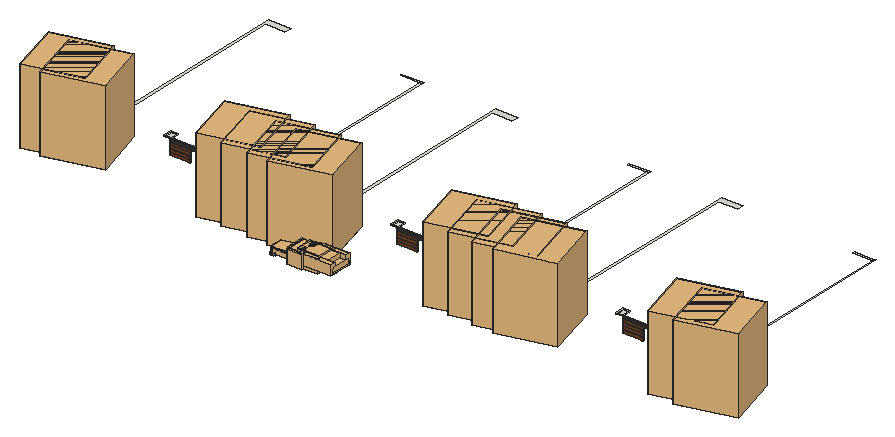
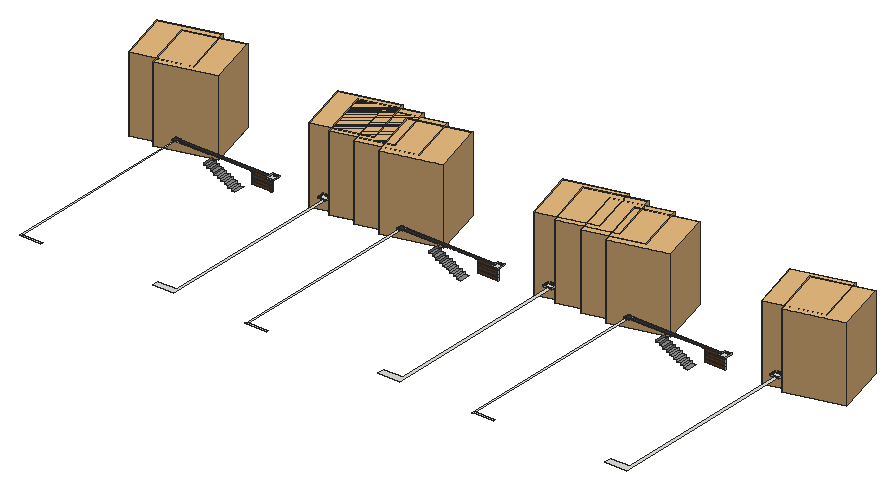
# SketchUp Ruby script. Lengths in inches.
U = 1.inch
M = Sketchup.active_model
def pt(a) = Geom::Point3d.new(a.map { |v| v * U })
def face(e, loops, mat)
  f = e.add_face(loops[0].map { |a| pt(a) })
  loops[1..].each { |l| e.add_face(l.map { |a| pt(a) }).erase! }
  f.material = f.back_material = mat if mat
  f
end
# faces: each face lists its corners as indices into pts; further lists are holes
def faces(e, pts, list, mat = nil) = list.each { |f| face(e, (f[0].is_a?(Array) ? f : [f]).map { |l| l.map { |i| pts[i] } }, mat) }
# xy, xz, yz: faces in a plane at the given z, y or x. An outline is a flat list of corners, or four numbers for a rectangle; further outlines are holes
def ring(l) = l.size == 4 ? [[l[0], l[1]], [l[2], l[1]], [l[2], l[3]], [l[0], l[3]]] : l.each_slice(2).to_a
def flat(e, list, mat, &to3) = list.each { |f| face(e, (f[0].is_a?(Array) ? f : [f]).map { |l| ring(l).map { |u, v| to3.(u, v) } }, mat) }
def xy(e, z, list, mat = nil) = flat(e, list, mat) { |x, y| [x, y, z] }
def xz(e, y, list, mat = nil) = flat(e, list, mat) { |x, z| [x, y, z] }
def yz(e, x, list, mat = nil) = flat(e, list, mat) { |y, z| [x, y, z] }
def lines(e, pts, list) = list.each { |a, b| e.add_line(pt(pts[a]), pt(pts[b])) }
# prism: a flat outline (further loops are holes) pulled along v
def prism(e, loops, v, mat = nil)
  f = face(e, loops, mat); d = Geom::Vector3d.new(v.map { |x| x * U })
  f.pushpull(f.normal.samedirection?(d) ? d.length : -d.length)
end
def box(e, o, s, mat = nil) = prism(e, [[o, [o[0] + s[0], o[1], o[2]], [o[0] + s[0], o[1] + s[1], o[2]], [o[0], o[1] + s[1], o[2]]]], [0, 0, s[2]], mat)
def at(x, y, z, deg = 0) = Geom::Transformation.translation(pt([x, y, z])) * Geom::Transformation.rotation(ORIGIN, Z_AXIS, deg.degrees)
def axes(o, x, y, z) = Geom::Transformation.new([*x, 0, *y, 0, *z, 0, *pt(o).to_a, 1])
def part(name) = M.definitions.add(name)
# library, detail: a bought-in or finely detailed component or shape, given as its bounding box
def library(name, o, s) = part(name).tap { |d| box(d.entities, o, s) }
def detail(e, o, s) = box(e.add_group.entities, o, s)
def put(e, d, t, mat = nil) = e.add_instance(d, t).tap { |i| i.material = mat if mat }
def group(e, t, mat = nil) = e.add_group.tap { |g| g.transformation = t; g.material = mat if mat }.entities
root = M.entities
M.materials.add("[0132_LightGray]").color = [169, 169, 169]
M.materials.add("[0136_Charcoal]").color = [17, 17, 17]
M.materials.add("[Blacktop Old 02]").color = [143, 145, 145]
M.materials.add("[Color M07]").color = [58, 58, 58]
M.materials.add("[Wood Veneer 01]").color = [120, 70, 37]
M.materials.add("s500 white").color = [237, 237, 230]
M.materials.add("s600").color = [22, 22, 22]
c1 = library("Group\#538",[0,0,0],[7.9,66.99,3.86])
c2 = library("Front car door",[0,0,0],[50.01,18.32,46.37])
c3 = library("Rear car door",[0,0,0],[51.74,11.92,46.37])
c4 = library("Palm tree \#1",[-4.09,-4.52,0],[193.52,193.51,258.93])
c5 = part("Palm+Tree")
put(c5.entities,c4,at(25.51,-21.81,0,15))
c6 = library("Group\#523",[0,0,0],[21.93,78.33,4.58])
c7 = library("Group\#520",[0,0,0],[63.89,71.13,20.26])
c8 = part("Group\#531")
p = [[17.05,0,0.12],[10.76,0.83,0.14],[10.77,0.78,0],[8.125,1.26,0.14],[7.82,1.25,0],[5.66,2.14,0],
  [5.93,2.16,0.13],[4.78,3.14,0.17],[4.32,3.23,0],[3.41,4.89,0],[3.73,4.98,0.17],[1.67,12.39,0],
  [2,12.39,0.17],[0,22.05,0],[0.34,21.8125,0.17],[1.49,22.05,0.22],[16.1,0.375,0.31],[17.15,0.01,0.31],
  [14.125,0.92,0.31],[11.23,1.28,0.31],[8.51,1.62,0.31],[5.54,2.89,0.31],[5.22,3.53,0.31],[4.82,5.07,0.31],
  [3.125,12.39,0.31],[1.65,21.85,0.31]]
faces(c8.entities,p,[[0,1,2],[2,3,4],[3,2,1],[5,4,6],[6,4,3],[7,8,5],[7,5,6],[9,7,10],
  [7,9,8],[11,9,12],[12,9,10],[13,11,14],[14,11,12],[14,15,13],[16,1,17],[1,0,17],
  [1,16,18],[19,3,1],[19,1,18],[3,20,6],[3,19,20],[6,20,21],[21,7,6],[22,7,21],
  [10,7,23],[22,23,7],[24,12,10],[23,24,10],[14,12,25],[24,25,12],[14,25,15]],"[0132_LightGray]")
c9 = library("Group\#541",[0,74.4,0],[63.33,6.34,17.85])
c10 = library("Component\#24",[0,0,0],[112.42,14.7,36.85])
c11 = library("Car headlight",[-0.14,0,-0.04],[12.61,20.03,8.76])
c12 = library("Group\#517",[0,0,0],[9.48,71.95,2.68])
c13 = library("Group\#529",[0,0,0],[27.27,66.27,16.46])
c14 = library("Group\#527",[0,0,0],[8.93,15.28,7.15])
c15 = library("Group\#519",[0,0,0],[35.29,74.27,19.26])
c16 = library("Group\#535",[-5.26,0,0],[129.69,69.79,18.37])
c17 = part("3D_Object__24")
g1 = group(c17.entities,at(-0.5,-39.39,30.52))
p = [[0.5,0,0],[0.5,0.09,0.49],[0.27,0.1875,0.49],[0.15,0.15,0.01],[0.85,0.15,0.01],[0.73,0.1875,0.49],
  [0.18,0.41,0.5],[0,0.5,0.02],[1,0.5,0.02],[0.82,0.41,0.5],[0.27,0.64,0.51],[0.15,0.85,0.04],
  [0.85,0.85,0.04],[0.73,0.64,0.51],[0.5,0.73,0.52],[0.5,1,0.04],[0.5,0.1,0.9],[0.33,0.17,0.9],
  [0.67,0.17,0.9],[0.26,0.34,0.91],[0.74,0.34,0.91],[0.33,0.5,0.91],[0.67,0.5,0.91],[0.5,0.57,0.91],
  [0.34,0.09,1.16],[0.5,0.03,1.16],[0.5,0.24,1.22],[0.66,0.09,1.16],[0.27,0.26,1.17],[0.73,0.26,1.17],
  [0.34,0.42,1.17],[0.5,0.48,1.17],[0.66,0.42,1.17]]
faces(g1,p,[[0,1,2,3],[4,5,1,0],[3,2,6,7],[8,9,5,4],[7,6,10,11],[12,13,9,8],[11,10,14,15],[15,14,13,12],
  [1,16,17,2],[1,5,18,16],[6,2,19],[17,19,2],[9,20,5],[18,5,20],[19,21,6],[20,9,22],
  [10,6,21],[13,22,9],[10,21,14],[23,14,21],[13,14,22],[23,22,14],[24,25,26],[25,27,26],
  [28,24,26],[27,29,26],[30,28,26],[31,30,26],[32,31,26],[29,32,26]])
g2 = group(c17.entities,at(-0.24,-39.37,31.42))
p = [[0.24,0.08,0],[0.24,0,0.26],[0.07,0.07,0.26],[0.07,0.14,0],[0.4,0.14,0],[0.4,0.07,0.26],
  [0.01,0.23,0.27],[0,0.31,0.01],[0.47,0.31,0.01],[0.46,0.23,0.27],[0.07,0.39,0.27],[0.07,0.48,0.01],
  [0.4,0.48,0.01],[0.4,0.39,0.27],[0.24,0.46,0.27],[0.24,0.54,0.01]]
faces(g2,p,[[0,1,2,3],[4,5,1,0],[3,2,6,7],[8,9,5,4],[7,6,10,11],[12,13,9,8],[11,10,14,15],[15,14,13,12]],"[0132_LightGray]")
c18 = library("Group\#540",[0,0,0],[73.87,53.92,3.7])
xy(root,13.04,[[998.26,300.25,1070.49,301],[1784.63,300.25,1856.87,301],[2565.01,300.25,2637.24,301]])
xy(root,17.875,[[1073.03,335.33,1085.03,371.33],[1859.4,335.33,1871.4,371.33],[2639.78,335.33,2651.78,371.33]],"[Blacktop Old 02]")
xy(root,22.41,[[998.26,300.25,1070.49,301],[1784.63,300.25,1856.87,301],[2565.01,300.25,2637.24,301]])
xy(root,23.79,[[998.26,300.25,1070.49,301],[1784.63,300.25,1856.87,301],[2565.01,300.25,2637.24,301]])
xy(root,23.875,[[1085.03,335.33,1097.03,371.33],[1871.4,335.33,1883.4,371.33],[2651.78,335.33,2663.78,371.33]],"[Blacktop Old 02]")
xy(root,29.875,[[1097.03,335.33,1109.03,371.33],[1883.4,335.33,1895.4,371.33],[2663.78,335.33,2675.78,371.33]],"[Blacktop Old 02]")
xy(root,33.16,[[998.26,300.25,1070.49,301],[1784.63,300.25,1856.87,301],[2565.01,300.25,2637.24,301]])
xy(root,34.54,[[998.26,300.25,1070.49,301],[1784.63,300.25,1856.87,301],[2565.01,300.25,2637.24,301]])
xy(root,35.875,[[1109.03,335.33,1121.03,371.33],[1895.4,335.33,1907.4,371.33],[2675.78,335.33,2687.78,371.33]],"[Blacktop Old 02]")
xy(root,41.875,[[1121.03,335.33,1133.03,371.33],[1907.4,335.33,1919.4,371.33],[2687.78,335.33,2699.78,371.33]],"[Blacktop Old 02]")
xy(root,43.91,[[998.26,300.25,1070.49,301],[1784.63,300.25,1856.87,301],[2565.01,300.25,2637.24,301]])
xy(root,45.29,[[998.26,300.25,1070.49,301],[1784.63,300.25,1856.87,301],[2565.01,300.25,2637.24,301]])
xy(root,47.875,[[1133.03,335.33,1145.03,371.33],[1919.4,335.33,1931.4,371.33],[2699.78,335.33,2711.78,371.33]],"[Blacktop Old 02]")
xy(root,53.875,[[1145.03,335.33,1157.03,371.33],[1931.4,335.33,1943.4,371.33],[2711.78,335.33,2723.78,371.33]],"[Blacktop Old 02]")
xy(root,54.66,[[1070.49,300.25,1216.78,301],[1219.26,300.25,1219.97,301],[1222.44,300.25,1223.16,301],[1225.63,300.25,1226.35,301],[1228.82,300.25,1229.53,301],
  [1232.01,300.25,1232.72,301],[1235.19,300.25,1235.91,301],[1238.38,300.25,1239.1,301],[1241.57,300.25,1242.28,301],[1244.76,300.25,1245.47,301],
  [1247.94,300.25,1248.66,301],[1251.13,300.25,1251.85,301],[1254.32,300.25,1255.03,301],[1257.51,300.25,1258.22,301],[1260.69,300.25,1261.41,301],
  [1263.88,300.25,1264.6,301],[1267.07,300.25,1267.78,301],[1270.26,300.25,1270.97,301],[1273.44,300.25,1274.16,301],[1276.63,300.25,1277.35,301],
  [1279.82,300.25,1280.53,301],[1283.01,300.25,1283.72,301],[1286.19,300.25,1286.85,301],[1289.32,300.25,1289.97,301],[1292.44,300.25,1293.1,301],
  [1295.57,300.25,1296.22,301],[1298.69,300.25,1299.35,301],[1301.82,300.25,1302.47,301],[1304.94,300.25,1305.6,301],[1308.07,300.25,1308.72,301],
  [1311.19,300.25,1311.85,301],[1314.32,300.25,1314.97,301],[1317.44,300.25,1318.1,301],[1856.87,300.25,2003.16,301],[2005.63,300.25,2006.35,301],
  [2008.82,300.25,2009.53,301],[2012.01,300.25,2012.72,301],[2015.19,300.25,2015.91,301],[2018.38,300.25,2019.1,301],[2021.57,300.25,2022.28,301],
  [2024.76,300.25,2025.47,301],[2027.94,300.25,2028.66,301],[2031.13,300.25,2031.85,301],[2034.32,300.25,2035.03,301],[2037.51,300.25,2038.22,301],
  [2040.69,300.25,2041.41,301],[2043.88,300.25,2044.6,301],[2047.07,300.25,2047.78,301],[2050.26,300.25,2050.97,301],[2053.44,300.25,2054.16,301],
  [2056.63,300.25,2057.35,301],[2059.82,300.25,2060.53,301],[2063.01,300.25,2063.72,301],[2066.19,300.25,2066.91,301],[2069.38,300.25,2070.1,301],
  [2072.57,300.25,2073.22,301],[2075.69,300.25,2076.35,301],[2078.82,300.25,2079.47,301],[2081.94,300.25,2082.6,301],[2085.07,300.25,2085.72,301],
  [2088.19,300.25,2088.85,301],[2091.32,300.25,2091.97,301],[2094.44,300.25,2095.1,301],[2097.57,300.25,2098.22,301],[2100.69,300.25,2101.35,301],
  [2103.82,300.25,2104.47,301],[2637.24,300.25,2783.53,301],[2786.01,300.25,2786.72,301],[2789.19,300.25,2789.91,301],[2792.38,300.25,2793.1,301],
  [2795.57,300.25,2796.28,301],[2798.76,300.25,2799.47,301],[2801.94,300.25,2802.66,301],[2805.13,300.25,2805.85,301],[2808.32,300.25,2809.03,301],
  [2811.51,300.25,2812.22,301],[2814.69,300.25,2815.41,301],[2817.88,300.25,2818.6,301],[2821.07,300.25,2821.78,301],[2824.26,300.25,2824.97,301],
  [2827.44,300.25,2828.16,301],[2830.63,300.25,2831.35,301],[2833.82,300.25,2834.53,301],[2837.01,300.25,2837.72,301],[2840.19,300.25,2840.91,301],
  [2843.38,300.25,2844.1,301],[2846.57,300.25,2847.28,301],[2849.76,300.25,2850.47,301],[2852.94,300.25,2853.6,301],[2856.07,300.25,2856.72,301],
  [2859.19,300.25,2859.85,301],[2862.32,300.25,2862.97,301],[2865.44,300.25,2866.1,301],[2868.57,300.25,2869.22,301],[2871.69,300.25,2872.35,301],
  [2874.82,300.25,2875.47,301],[2877.94,300.25,2878.6,301],[2881.07,300.25,2881.72,301],[2884.19,300.25,2884.85,301]])
xy(root,58.8125,[[1328.59,315.3125,1334.59,969.375],[2114.96,315.3125,2120.96,969.375],[2895.34,315.3125,2901.34,969.375],[1260.59,969.375,1328.59,975.9375],[1328.59,969.375,1334.59,975.9375],
  [2046.96,969.375,2114.96,975.9375],[2114.96,969.375,2120.96,975.9375],[2827.34,969.375,2895.34,975.9375],[2895.34,969.375,2901.34,975.9375]])
xy(root,59.875,[[1157.03,335.33,1169.03,371.33],[1943.4,335.33,1955.4,371.33],[2723.78,335.33,2735.78,371.33]],"[Blacktop Old 02]")
xy(root,62.25,[[1318.09,298.8125,1320.28,300.25],[1320.28,298.8125,1334.59,301],[1334.59,298.8125,1336.78,301],[2104.46,298.8125,2106.65,300.25],[2106.65,298.8125,2120.96,301],
  [2120.96,298.8125,2123.15,301],[2884.84,298.8125,2887.03,300.25],[2887.03,298.8125,2901.34,301],[2901.34,298.8125,2903.53,301],[1318.09,300.25,1320.28,308.75],
  [2104.46,300.25,2106.65,308.75],[2884.84,300.25,2887.03,308.75],[1320.28,301,1334.59,315.3125],[1334.59,301,1336.78,315.3125],[2106.65,301,2120.96,315.3125],
  [2120.96,301,2123.15,315.3125],[2887.03,301,2901.34,315.3125],[2901.34,301,2903.53,315.3125],[1318.09,308.75,1320.28,315.3125],[2104.46,308.75,2106.65,315.3125],
  [2884.84,308.75,2887.03,315.3125]])
xy(root,62.25,[[998.26,300.25,1318.09,308.75],[1784.63,300.25,2104.46,308.75],[2565.01,300.25,2884.84,308.75]],"[Color M07]")
xy(root,64.4375,[[1318.09,298.8125,1336.78,315.3125],[2104.46,298.8125,2123.15,315.3125],[2884.84,298.8125,2903.53,315.3125]],"[Color M07]")
xy(root,65.875,[[796.71,297,800.71,301],[800.71,297,823.45,301],[823.45,297,827.45,301],[1583.09,297,1587.09,301],[1587.09,297,1609.83,301],
  [1609.83,297,1613.83,301],[2363.46,297,2367.46,301],[2367.46,297,2390.2,301],[2390.2,297,2394.2,301],[978.32,297.1875,1002.07,301],
  [1764.69,297.1875,1788.44,301],[2545.07,297.1875,2568.82,301],[796.71,301,800.71,321.97],[800.71,301,823.45,321.97],[823.45,301,827.45,321.97],
  [978.32,301,982.13,327.09],[982.13,301,998.26,327.09],[998.26,301,1002.07,327.09],[1583.09,301,1587.09,321.97],[1587.09,301,1609.83,321.97],
  [1609.83,301,1613.83,321.97],[1764.69,301,1768.51,327.09],[1768.51,301,1784.63,327.09],[1784.63,301,1788.44,327.09],[2363.46,301,2367.46,321.97],
  [2367.46,301,2390.2,321.97],[2390.2,301,2394.2,321.97],[2545.07,301,2548.88,327.09],[2548.88,301,2565.01,327.09],[2565.01,301,2568.82,327.09],
  [800.71,321.97,808.46,321.97,808.46,952.09,874.71,952.09,874.71,975.9375,800.71,975.9375],[1587.09,321.97,1594.84,321.97,1594.84,952.09,1661.09,952.09,1661.09,975.9375,1587.09,975.9375],[2367.46,321.97,2375.21,321.97,2375.21,952.09,2441.46,952.09,2441.46,975.9375,2367.46,975.9375]])
xy(root,65.875,[[1169.03,335.33,1181.03,371.33],[1955.4,335.33,1967.4,371.33],[2735.78,335.33,2747.78,371.33]],"[Blacktop Old 02]")
xz(root,297,[[796.71,65.875,827.45,69.625],[1583.09,65.875,1613.83,69.625],[2363.46,65.875,2394.2,69.625]],"[Color M07]")
xz(root,297.1875,[[978.32,65.875,1002.07,69.625],[1764.69,65.875,1788.44,69.625],[2545.07,65.875,2568.82,69.625]])
xz(root,298.8125,[[1318.09,62.25,1336.78,64.4375],[2104.46,62.25,2123.15,64.4375],[2884.84,62.25,2903.53,64.4375]],"[Color M07]")
xz(root,300.25,[[998.26,54.66,1320.28,62.25],[1784.63,54.66,2106.65,62.25],[2565.01,54.66,2887.03,62.25]],"[Color M07]")
xz(root,300.25,[[998.26,13.04,1070.49,22.41],[1784.63,13.04,1856.87,22.41],[2565.01,13.04,2637.24,22.41],[998.26,23.79,1070.49,33.16],[1784.63,23.79,1856.87,33.16],
  [2565.01,23.79,2637.24,33.16],[998.26,34.54,1070.49,43.91],[1784.63,34.54,1856.87,43.91],[2565.01,34.54,2637.24,43.91],[998.26,45.29,1070.49,54.66],
  [1784.63,45.29,1856.87,54.66],[2565.01,45.29,2637.24,54.66]],"[Wood Veneer 01]")
xz(root,301,[[998.26,22.41,1070.49,23.79],[1784.63,22.41,1856.87,23.79],[2565.01,22.41,2637.24,23.79],[998.26,33.16,1070.49,34.54],[1784.63,33.16,1856.87,34.54],
  [2565.01,33.16,2637.24,34.54],[998.26,43.91,1070.49,45.29],[1784.63,43.91,1856.87,45.29],[2565.01,43.91,2637.24,45.29]],"[Wood Veneer 01]")
xz(root,315.3125,[[1318.09,62.25,1320.28,64.4375],[1320.28,62.25,1334.59,64.4375],[1334.59,62.25,1336.78,64.4375],[2104.46,62.25,2106.65,64.4375],[2106.65,62.25,2120.96,64.4375],
  [2120.96,62.25,2123.15,64.4375],[2884.84,62.25,2887.03,64.4375],[2887.03,62.25,2901.34,64.4375],[2901.34,62.25,2903.53,64.4375]])
xz(root,321.97,[[796.71,65.875,800.71,69.625],[800.71,65.875,808.46,69.625],[808.46,65.875,823.45,69.625],[823.45,65.875,827.45,69.625],[1583.09,65.875,1587.09,69.625],
  [1587.09,65.875,1594.84,69.625],[1594.84,65.875,1609.83,69.625],[1609.83,65.875,1613.83,69.625],[2363.46,65.875,2367.46,69.625],[2367.46,65.875,2375.21,69.625],
  [2375.21,65.875,2390.2,69.625],[2390.2,65.875,2394.2,69.625]])
xz(root,327.09,[[978.32,65.875,1002.07,69.625],[1764.69,65.875,1788.44,69.625],[2545.07,65.875,2568.82,69.625]])
yz(root,796.71,[[297,65.875,301,69.625],[301,65.875,321.97,69.625]])
yz(root,827.45,[[297,65.875,321.97,69.625]],"[Color M07]")
yz(root,978.32,[[297.1875,65.875,327.09,69.625]])
yz(root,998.26,[[300.25,13.04,301,22.41],[300.25,23.79,301,33.16],[300.25,34.54,301,43.91],[300.25,45.29,301,54.66],[300.25,54.66,301,62.25]])
yz(root,1002.07,[[297.1875,65.875,327.09,69.625]])
yz(root,1070.49,[[300.25,13.04,301,22.41],[300.25,23.79,301,33.16],[300.25,34.54,301,43.91],[300.25,45.29,301,54.66]])
yz(root,1085.03,[[335.33,17.875,371.33,23.875]])
yz(root,1097.03,[[335.33,23.875,371.33,29.875]])
yz(root,1109.03,[[335.33,29.875,371.33,35.875]])
yz(root,1121.03,[[335.33,35.875,371.33,41.875]])
yz(root,1133.03,[[335.33,41.875,371.33,47.875]])
yz(root,1145.03,[[335.33,47.875,371.33,53.875]],"[Blacktop Old 02]")
yz(root,1157.03,[[335.33,53.875,371.33,59.875]],"[Blacktop Old 02]")
yz(root,1169.03,[[335.33,59.875,371.33,65.875]],"[Blacktop Old 02]")
yz(root,1181.03,[[335.33,65.875,371.33,71.875]],"[Blacktop Old 02]")
yz(root,1318.09,[[298.8125,62.25,301,64.4375],[301,62.25,308.75,64.4375],[308.75,62.25,315.3125,64.4375]])
yz(root,1320.28,[[300.25,54.66,301,62.25]])
yz(root,1336.78,[[298.8125,62.25,315.3125,64.4375]])
yz(root,1583.09,[[297,65.875,301,69.625],[301,65.875,321.97,69.625]])
yz(root,1613.83,[[297,65.875,321.97,69.625]],"[Color M07]")
yz(root,1764.69,[[297.1875,65.875,327.09,69.625]])
yz(root,1784.63,[[300.25,13.04,301,22.41],[300.25,23.79,301,33.16],[300.25,34.54,301,43.91],[300.25,45.29,301,54.66],[300.25,54.66,301,62.25]])
yz(root,1788.44,[[297.1875,65.875,327.09,69.625]])
yz(root,1856.87,[[300.25,13.04,301,22.41],[300.25,23.79,301,33.16],[300.25,34.54,301,43.91],[300.25,45.29,301,54.66]])
yz(root,1871.4,[[335.33,17.875,371.33,23.875]])
yz(root,1883.4,[[335.33,23.875,371.33,29.875]])
yz(root,1895.4,[[335.33,29.875,371.33,35.875]])
yz(root,1907.4,[[335.33,35.875,371.33,41.875]])
yz(root,1919.4,[[335.33,41.875,371.33,47.875]])
yz(root,1931.4,[[335.33,47.875,371.33,53.875]],"[Blacktop Old 02]")
yz(root,1943.4,[[335.33,53.875,371.33,59.875]],"[Blacktop Old 02]")
yz(root,1955.4,[[335.33,59.875,371.33,65.875]],"[Blacktop Old 02]")
yz(root,1967.4,[[335.33,65.875,371.33,71.875]],"[Blacktop Old 02]")
yz(root,2104.46,[[298.8125,62.25,301,64.4375],[301,62.25,308.75,64.4375],[308.75,62.25,315.3125,64.4375]])
yz(root,2106.65,[[300.25,54.66,301,62.25]])
yz(root,2123.15,[[298.8125,62.25,315.3125,64.4375]])
yz(root,2363.46,[[297,65.875,301,69.625],[301,65.875,321.97,69.625]])
yz(root,2394.2,[[297,65.875,321.97,69.625]],"[Color M07]")
yz(root,2545.07,[[297.1875,65.875,327.09,69.625]])
yz(root,2565.01,[[300.25,13.04,301,22.41],[300.25,23.79,301,33.16],[300.25,34.54,301,43.91],[300.25,45.29,301,54.66],[300.25,54.66,301,62.25]])
yz(root,2568.82,[[297.1875,65.875,327.09,69.625]])
yz(root,2637.24,[[300.25,13.04,301,22.41],[300.25,23.79,301,33.16],[300.25,34.54,301,43.91],[300.25,45.29,301,54.66]])
yz(root,2651.78,[[335.33,17.875,371.33,23.875]])
yz(root,2663.78,[[335.33,23.875,371.33,29.875]])
yz(root,2675.78,[[335.33,29.875,371.33,35.875]])
yz(root,2687.78,[[335.33,35.875,371.33,41.875]])
yz(root,2699.78,[[335.33,41.875,371.33,47.875]])
yz(root,2711.78,[[335.33,47.875,371.33,53.875]],"[Blacktop Old 02]")
yz(root,2723.78,[[335.33,53.875,371.33,59.875]],"[Blacktop Old 02]")
yz(root,2735.78,[[335.33,59.875,371.33,65.875]],"[Blacktop Old 02]")
yz(root,2747.78,[[335.33,65.875,371.33,71.875]],"[Blacktop Old 02]")
yz(root,2884.84,[[298.8125,62.25,301,64.4375],[301,62.25,308.75,64.4375],[308.75,62.25,315.3125,64.4375]])
yz(root,2887.03,[[300.25,54.66,301,62.25]])
yz(root,2903.53,[[298.8125,62.25,315.3125,64.4375]])
p = [[1609.83,301,65.875],[1609.83,301,69.625],[1587.09,301,65.875],[1587.09,301,69.625],[2120.96,301,62.25],[2120.96,301,64.4375],
  [2106.65,301,62.25],[2106.65,301,64.4375],[1334.59,301,62.25],[1334.59,301,64.4375],[1320.28,301,62.25],[1320.28,301,64.4375],
  [823.45,301,65.875],[823.45,301,69.625],[800.71,301,65.875],[800.71,301,69.625],[2901.34,301,62.25],[2901.34,301,64.4375],
  [2887.03,301,62.25],[2887.03,301,64.4375],[2390.2,301,65.875],[2390.2,301,69.625],[2367.46,301,65.875],[2367.46,301,69.625],
  [1563.23,111.57,28.09],[1563.23,111.57,28.14],[1586.57,68.48,18.05],[1586.71,68.49,18.18],[1586.57,30.29,18.05],[1586.71,30.3,18.18]]
lines(root,p,[[0,1],[2,3],[4,5],[6,7],[8,9],[10,11],[12,13],[14,15],[16,17],[18,19],[20,21],[22,23],
  [24,25],[26,27],[28,29]])
put(root,c1,at(1554.57,41.71,12.39),"s600")
put(root,c2,at(1620.37,102.88,12.875))
put(root,c3,axes([1667.84,47.52,12.875],[1,0,0],[0,-1,0],[0,0,1]),"s600")
put(root,c2,axes([1620.37,47.52,12.875],[1,0,0],[0,-1,0],[0,0,1]))
put(root,c3,at(1667.84,102.88,12.875),"s600")
put(root,c5,at(1493.92,99.07,18.26))
put(root,c5,at(1423.92,99.07,18.26))
put(root,c5,at(2033.23,99.07,18.26))
put(root,c5,at(2119.29,99.07,18.26))
put(root,c5,at(1332.92,99.07,18.26))
put(root,c5,at(1246.85,99.07,18.26))
put(root,c5,at(637.54,99.07,18.26))
put(root,c5,at(707.54,99.07,18.26))
put(root,c5,at(2813.6,99.07,18.26))
put(root,c5,at(2899.67,99.07,18.26))
put(root,c5,at(2274.29,99.07,18.26))
put(root,c5,at(2204.29,99.07,18.26))
put(root,c6,at(1553.45,36.04,18.9))
put(root,c7,at(1556.41,39.63,22.32))
put(root,c8,axes([1557.49,114.3,23.17],[1,0,0],[0,-1,0],[0,0,1]),"s600")
put(root,c8,at(1557.49,36.09,23.17),"s600")
g3 = group(root,at(1559.15,41.17,23.48))
p = [[1.7,7.17,1.16],[1.47,7.32,0],[3.4,0,1.16],[3.17,0,0],[0.28,16.38,1.16],[0,16.77,0],
  [0.28,51.68,1.16],[1.47,60.75,0],[0,51.29,0],[1.7,60.89,1.16],[3.4,68.07,1.16],[3.17,68.06,0]]
faces(g3,p,[[0,1,2],[3,2,1],[4,1,0],[1,4,5],[6,7,8],[7,6,9],[7,9,10],[10,11,7]],"s500 white")
put(root,c9,at(1562.32,34.83,23.48))
put(root,c9,axes([1562.32,115.57,23.48],[1,0,0],[0,-1,0],[0,0,1]))
put(root,c10,axes([1655.4,115.12,23.55],[1,0,0],[0,-1,0],[0,0,1]))
put(root,c10,at(1655.4,35.28,23.55))
put(root,c11,at(1559.41,37.52,23.92))
put(root,c11,axes([1559.41,112.88,23.92],[1,0,0],[0,-1,0],[0,0,1]))
g4 = group(root,at(1767.58,42.5625,26.3125))
yz(g4,0.6,[[14.08,0,32.64,0.73,14.08,0.73],[51.2,0,51.2,0.73,32.64,0.73]],"s500 white")
p = [[0,0,0.73],[0.6,14.08,0],[0.6,14.08,0.73],[0,0,0],[0.6,32.64,0.73],[0.63,32.64,0],
  [0.6,51.2,0],[0,65.27,0.73],[0.6,51.2,0.73],[0,65.27,0]]
faces(g4,p,[[0,1,2],[1,0,3],[4,1,5],[6,4,5],[6,7,8],[7,6,9]],"s500 white")
put(root,c12,at(1758.73,39.22,27.05),"s600")
put(root,c13,at(1740.85,42.07,29.02))
put(root,c14,at(1759.16,39.25,29.73),"s600")
put(root,c14,axes([1759.16,111.15,29.73],[1,0,0],[0,-1,0],[0,0,1]),"s600")
put(root,c15,at(1620.94,38.0625,40.77))
put(root,c16,at(1619.5,40.3,40.83),"s600")
g5 = group(root,at(1613.57,40.22,40.83),"s600")
p = [[6.73,0,0.1],[6.125,2.06,0.02],[5.51,2.32,0.36],[7.04,0.08,0],[4.43,4.6,0.63],[5.38,4.27,0.11],
  [4.43,65.35,0.63],[6.125,67.89,0.02],[5.51,67.63,0.36],[5.38,65.68,0.11],[6.73,69.95,0.1],[7.04,69.87,0],
  [3.54,11.56,0.11],[2.8125,11.41,1.02],[1.48,18.64,1.39],[2.14,18.85,0.5],[3.54,58.39,0.11],[1.48,51.3125,1.39],
  [2.14,51.1,0.5],[2.8125,58.54,1.02],[1.16,26.91,0.5],[0.49,26.81,1.67],[0,34.98,1.75],[0.68,34.98,0.5],
  [1.16,43.04,0.5],[0.49,43.14,1.67]]
faces(g5,p,[[0,1,2],[1,0,3],[1,4,2],[4,1,5],[6,7,8],[7,6,9],[7,10,8],[10,7,11],
  [12,4,5],[4,12,13],[12,14,13],[14,12,15],[16,17,18],[17,16,19],[16,6,19],[6,16,9],
  [14,20,21],[20,14,15],[20,22,21],[22,20,23],[24,22,23],[22,24,25],[24,17,25],[17,24,18]],"[0136_Charcoal]")
g6 = group(root,at(1724.89,112.41,41.2))
p = [[-4.62,-0.38,0.17],[-4.46,-0.3,-0.05],[-3.5,-0.34,-0.04],[-3.5,-0.35,-0.03],[-4.03,-0.5,0.4],[-4.12,-0.54,0.49],
  [-4.15,-0.57,0.58],[-4.125,-0.6,0.65],[-4.06,-0.62,0.7],[-3.96,-0.64,0.73],[-3.83,-0.65,0.74],[-3.73,-0.65,0.74],
  [-3.62,-0.65,0.72],[-3.62,-0.73,0.92],[-3.77,-0.73,0.94],[-3.93,-0.73,0.95],[-4.05,-0.72,0.94],[-4.17,-0.71,0.92],
  [-4.27,-0.69,0.89],[-4.35,-0.67,0.85],[-4.42,-0.65,0.81],[-4.47,-0.625,0.75],[-4.5,-0.6,0.69],[-4.51,-0.57,0.625],
  [-4.48,-0.52,0.5],[-4.38,-0.48,0.38],[-4.15,-0.41,0.17],[-4.61,0.11,0.47],[-4.45,0.1875,0.25],[-3.49,0.15,0.26],
  [-2.36,-0.8,0.96],[-1.4,-0.4375,-0.03],[-0.96,-0.46,-0.02],[-0.06,-0.9,0.98],[-0.68,-0.87,0.97],[-1.19,-0.6,0.36],
  [-1.74,-0.82,0.96],[-0.95,0.03,0.28],[-0.05,-0.41,1.28],[-2.96,-0.37,-0.04],[-2.63,-0.38,-0.04],[-2.64,-0.62,0.56],
  [-2.52,-0.61,0.51],[-2.38,-0.6,0.48],[-2.39,-0.69,0.7],[-2.49,-0.7,0.75],[-2.58,-0.72,0.8],[-2.65,-0.74,0.86],
  [-2.71,-0.77,0.93],[-2.98,-0.76,0.93],[-2.97,-0.27,1.23],[-2.95,0.125,0.26],[-2.35,-0.3,1.26],[-1.39,0.05,0.27],
  [-2.62,0.11,0.27],[-2.63,-0.13,0.86],[-3.49,0.14,0.27],[-4.02,-0.01,0.71],[-4.37,0.01,0.68],[-4.14,0.09,0.48],
  [-1.73,-0.33,1.27],[-1.18,-0.11,0.67],[-0.67,-0.38,1.27],[-2.7,-0.28,1.23],[-2.64,-0.25,1.16],[-2.57,-0.23,1.1],
  [-2.48,-0.21,1.05],[-2.375,-0.2,1],[-2.37,-0.11,0.78],[-2.5,-0.12,0.8125],[-4.47,-0.03,0.8],[-4.5,-0.08,0.93],
  [-4.49,-0.11,0.99],[-4.46,-0.13,1.05],[-4.41,-0.16,1.11],[-4.34,-0.18,1.16],[-4.25,-0.2,1.2],[-4.15,-0.22,1.22],
  [-4.04,-0.23,1.24],[-3.92,-0.24,1.25],[-3.76,-0.24,1.24],[-3.61,-0.24,1.23],[-3.61,-0.16,1.02],[-3.72,-0.16,1.04],
  [-3.82,-0.16,1.05],[-3.95,-0.15,1.03],[-4.05,-0.13,1],[-4.11,-0.11,0.95],[-4.14,-0.08,0.88],[-4.11,-0.04,0.8]]
faces(g6,p,[[0,1,2,3,4,5,6,7,8,9,10,11,12,13,14,15,16,17,18,19,20,21,22,23,24,25,26],[1,0,27,28],[2,1,28,29],[30,31,32,33,34,35,36],[33,32,37,38],[39,40,41,42,43,44,45,46,47,48,49],[39,49,50,51],[31,30,52,53],
  [41,40,54,55],[4,3,56,57],[32,31,53,37],[40,39,51,54],[3,2,29,56],[26,25,58,59],[0,26,59,27],[53,52,60,61,62,38,37],
  [54,51,50,63,64,65,66,67,68,69,55],[28,27,59,58,70,71,72,73,74,75,76,77,78,79,80,81,82,83,84,85,86,87,88,89,57,56,29],[35,34,62,61],[36,35,61,60],[25,24,70,58],[5,4,57,89],[44,43,68,67],[24,23,71,70],
  [6,5,89,88],[42,41,55,69],[43,42,69,68],[23,22,72,71],[7,6,88,87],[8,7,87,86],[11,10,84,83],[12,11,83,82],
  [13,12,82,81],[46,45,66,65],[45,44,67,66],[22,21,73,72],[9,8,86,85],[10,9,85,84],[20,19,75,74],[47,46,65,64],
  [21,20,74,73],[49,48,63,50],[48,47,64,63],[19,18,76,75],[18,17,77,76],[17,16,78,77],[16,15,79,78],[15,14,80,79],
  [14,13,81,80],[34,33,38,62],[30,36,60,52]],"[0132_LightGray]")
g7 = group(root,at(1722.07,37.94,41.125))
prism(g7,[[[2.93,0.74,0.01],[2.6,0.73,0.02],[2.59,0.95,0.63],[2.47,0.93,0.59],[2.34,0.91,0.55],[2.34,1,0.78],[2.44,1.02,0.83],[2.53,1.04,0.88],[2.6,1.07,0.95],[2.65,1.1,1.02],[2.92,1.1,1.01]]],[0.02,-0.67,0.25],"[0132_LightGray]")
prism(g7,[[[4.58,0.875,0.23],[4.43,0.79,0],[3.47,0.76,0.01],[3.47,0.76,0.02],[3.99,0.94,0.47],[4.07,0.98,0.57],[4.1,1.01,0.65],[4.08,1.04,0.73],[4.01,1.06,0.78],[3.91,1.07,0.8125],[3.78,1.07,0.83],[3.68,1.06,0.82],[3.57,1.05,0.8],[3.57,1.13,1.01],[3.72,1.14,1.03],[3.87,1.15,1.04],[4,1.15,1.03],[4.11,1.15,1.01],[4.21,1.14,0.98],[4.3,1.125,0.94],[4.37,1.11,0.89],[4.42,1.09,0.83],[4.45,1.07,0.77],[4.47,1.05,0.7],[4.43,1,0.57],[4.34,0.95,0.45],[4.12,0.86,0.23]]],[0.02,-0.67,0.25],"[0132_LightGray]")
prism(g7,[[[2.3,1.1,1.05],[1.37,0.6875,0.03],[0.93,0.67,0.03],[0,1.02,1.07],[0.62,1.04,1.0625],[1.15,0.83,0.43],[1.68,1.08,1.05]]],[0.02,-0.67,0.25],"[0132_LightGray]")
g8 = group(root,at(1765.98,43.4375,41.79),"s600")
prism(g8,[[[0.58,63.0625,0.1],[0.55,62.99,0.11],[0.51,62.93,0.13],[0.45,62.89,0.14],[0.375,62.86,0.15],[0.3,62.85,0.15],[0.22,62.86,0.15],[0.15,62.88,0.14],[0.09,62.93,0.13],[0.04,62.99,0.12],[0.01,63.06,0.1],[0,63.13,0.08],[0.01,63.2,0.06],[0.04,63.27,0.04],[0.08,63.33,0.02],[0.14,63.38,0.01],[0.22,63.41,0],[0.29,63.42,0],[0.37,63.41,0],[0.44,63.38,0.01],[0.5,63.34,0.02],[0.55,63.28,0.04],[0.58,63.21,0.06],[0.59,63.14,0.08]]],[0,0.1,0.38],"[0132_LightGray]")
prism(g8,[[[0.55,0.53,0.11],[0.58,0.46,0.1],[0.59,0.38,0.08],[0.58,0.31,0.06],[0.55,0.24,0.04],[0.5,0.18,0.02],[0.44,0.14,0.01],[0.37,0.11,0],[0.29,0.1,0],[0.22,0.11,0],[0.14,0.14,0.01],[0.08,0.1875,0.02],[0.04,0.25,0.04],[0.01,0.32,0.06],[0,0.39,0.08],[0.01,0.46,0.1],[0.04,0.53,0.12],[0.09,0.59,0.13],[0.15,0.64,0.14],[0.22,0.66,0.15],[0.3,0.67,0.15],[0.375,0.66,0.15],[0.45,0.63,0.14],[0.51,0.59,0.13]]],[0,-0.1,0.38],"[0132_LightGray]")
put(root,c17,axes([1743.57,90.91,-11.0625],[1.29,0,0],[0,1.29,0],[0,0,1.77735]),"s600")
g9 = group(root,at(1740.85,75.2,44.4),"s600")
p = [[1.77,27.6,0.3125],[0.24,32.57,0.13],[0,32.46,0],[2.08,27.64,0.49],[2.87,20.64,0.73],[2.55,20.64,0.58],
  [3.26,11.29,0.94],[3,11.29,0.84],[3.39,0,1.09],[3.08,0,0.92]]
faces(g9,p,[[0,1,2],[1,0,3],[0,4,3],[4,0,5],[6,5,7],[5,6,4],[7,8,6],[8,7,9]])
g10 = group(root,at(1713.09,42.07,44.4))
p = [[28,0.57,0.13],[27.76,0.67,0],[19.65,2.125,4.48],[27.76,65.59,0],[28,65.7,0.13],[19.65,64.14,4.48],
  [19.86,2.01,4.34],[27.79,0,0.09],[20.18,1.33,4],[19.86,64.25,4.34],[20.18,64.93,4],[27.79,66.27,0.09],
  [14.65,2.55,6.89],[14.65,63.72,6.89],[14.53,3.2,7.125],[14.53,63.0625,7.125],[14.29,3.3,7.125],[14.29,62.96,7.125],
  [8.96,4.58,10.03],[9.12,3.9,9.78],[8.96,61.6875,10.03],[9.12,62.37,9.78],[8.75,4.68,10.03],[8.75,61.59,10.03],
  [4.71,5.02,11.96],[4.71,61.25,11.96],[4.8,5.69,12.05],[4.59,5.81,12.05],[4.8,60.57,12.05],[4.59,60.46,12.05],
  [0,6.3,14.13],[0.33,6.78,14],[0.44,6.82,13.9375],[0.44,59.45,13.9375],[0.33,59.49,14],[0,59.97,14.13]]
faces(g10,p,[[0,1,2],[3,4,5],[0,6,7],[6,8,7],[0,2,6],[5,4,9],[10,9,11],[9,4,11],
  [6,12,8],[13,9,10],[12,6,14],[2,14,6],[9,13,15],[15,5,9],[14,2,16],[5,15,17],
  [18,12,14],[12,18,19],[13,20,15],[20,13,21],[16,18,14],[18,16,22],[17,20,23],[20,17,15],
  [18,24,19],[25,20,21],[24,18,26],[22,26,18],[26,22,27],[23,28,29],[20,25,28],[28,23,20],
  [26,30,24],[30,26,31],[27,31,26],[27,32,31],[33,29,34],[28,35,34],[34,29,28],[35,28,25]],"[0136_Charcoal]")
g11 = group(root,at(1740.85,42.63,44.4),"s600")
p = [[0.24,0,0.13],[1.77,4.96,0.3125],[0,0.11,0],[2.08,4.93,0.49],[2.87,11.92,0.73],[2.55,11.92,0.58],
  [3.26,21.27,0.94],[3,21.27,0.84],[3.39,32.57,1.09],[3.08,32.57,0.92]]
faces(g11,p,[[0,1,2],[1,0,3],[4,1,3],[1,4,5],[6,5,4],[5,6,7],[8,7,6],[7,8,9]])
put(root,c18,at(1641.12,48.24,57.76))
g12 = group(root,at(1653.44,52.99,60.22))
p = [[0.32,2.1875,0.18],[7.39,3.76,0.59],[-0.4,2.38,0.15],[-0.93,2.91,0.125],[-1.12,3.625,0.16],[-0.93,41.52,0.125],
  [-1.12,40.8,0.16],[7.39,40.67,0.59],[-0.4,42.05,0.15],[0.32,42.24,0.18],[7.63,2.1875,0.45],[6.64,10.92,0.99],
  [-1.12,10.92,0.7],[-1.12,33.51,0.7],[6.64,33.51,0.99],[7.63,42.24,0.45],[16.47,2.1875,0.53],[16.47,42.24,0.53],
  [17.1875,2.38,0.55],[17.72,2.91,0.59],[17.1875,42.05,0.55],[17.72,41.52,0.59],[17.91,3.63,0.63],[17.91,10.92,1.1],
  [17.91,40.8,0.63],[17.91,33.51,1.1],[6.17,22.21,1.12],[-1.12,22.21,0.92],[17.91,22.21,1.22]]
faces(g12,p,[[0,1,2],[3,2,1],[4,3,1],[5,6,7],[8,5,7],[7,9,8],[1,0,10],[1,11,4],
  [12,4,11],[6,13,14],[14,7,6],[9,7,15],[10,16,1],[17,15,7],[1,19,22],[11,22,23],
  [11,1,22],[7,14,24],[24,14,25],[21,7,24],[26,27,12],[26,12,11],[27,26,13],[13,26,14],
  [26,11,23],[14,26,25],[26,23,28],[25,26,28]],"s500 white")
faces(g12,p,[[18,1,16],[1,18,19],[20,7,21],[7,20,17]])
